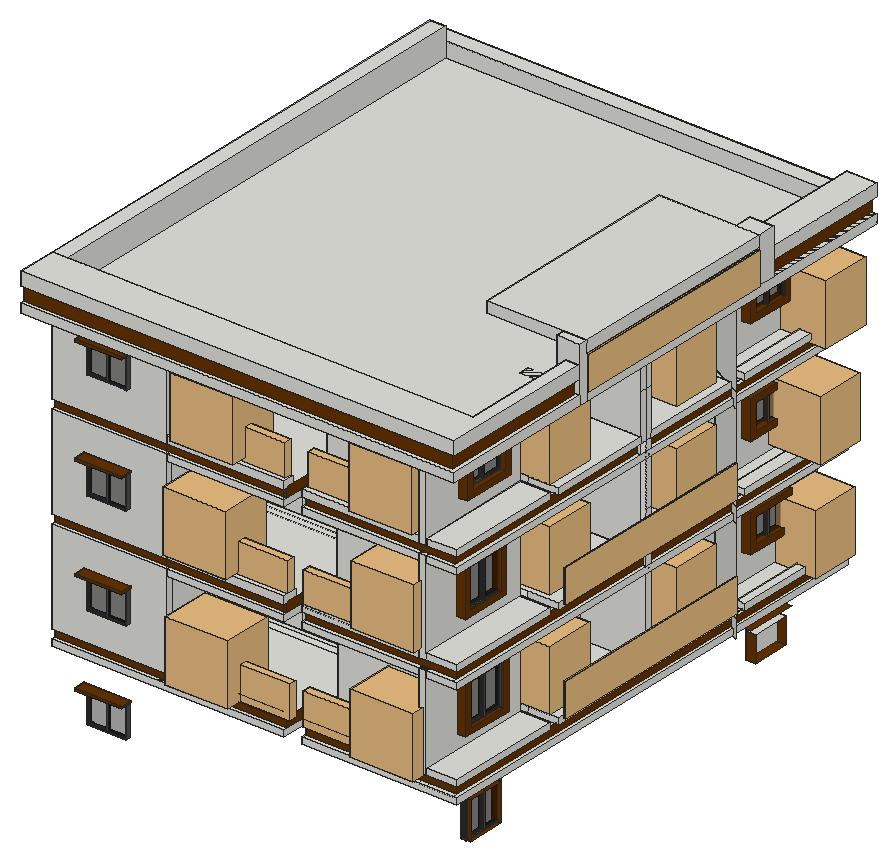
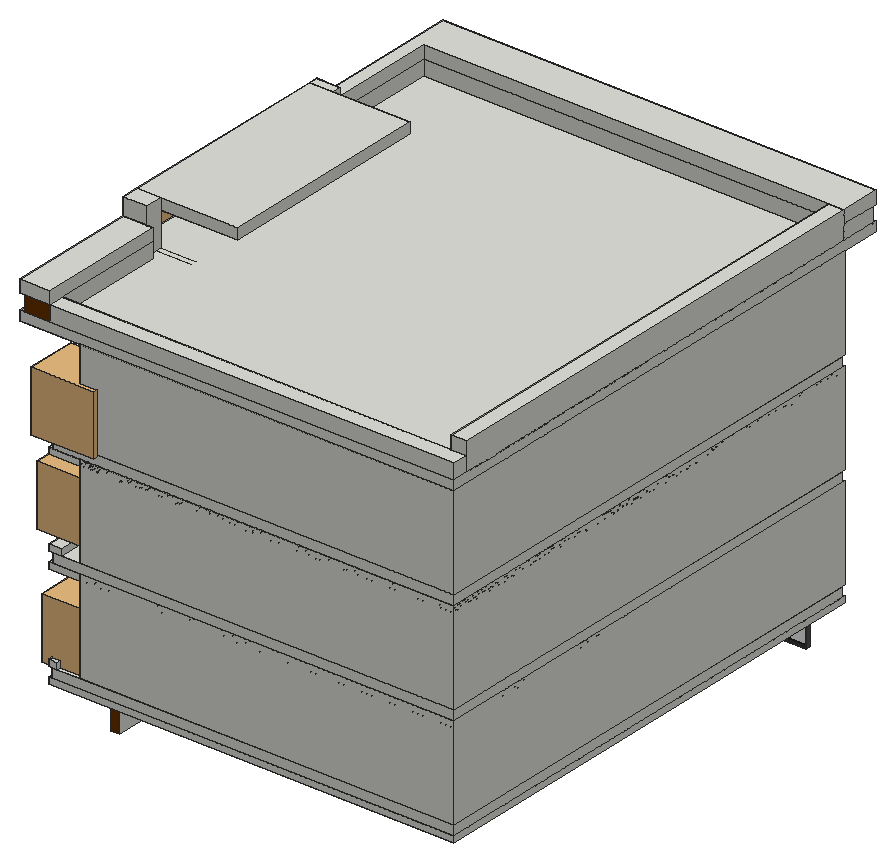
# SketchUp Ruby script. Lengths in inches.
U = 1.inch
M = Sketchup.active_model
def pt(a) = Geom::Point3d.new(a.map { |v| v * U })
def face(e, loops, mat)
  f = e.add_face(loops[0].map { |a| pt(a) })
  loops[1..].each { |l| e.add_face(l.map { |a| pt(a) }).erase! }
  f.material = f.back_material = mat if mat
  f
end
# faces: each face lists its corners as indices into pts; further lists are holes
def faces(e, pts, list, mat = nil) = list.each { |f| face(e, (f[0].is_a?(Array) ? f : [f]).map { |l| l.map { |i| pts[i] } }, mat) }
# xy, xz, yz: faces in a plane at the given z, y or x. An outline is a flat list of corners, or four numbers for a rectangle; further outlines are holes
def ring(l) = l.size == 4 ? [[l[0], l[1]], [l[2], l[1]], [l[2], l[3]], [l[0], l[3]]] : l.each_slice(2).to_a
def flat(e, list, mat, &to3) = list.each { |f| face(e, (f[0].is_a?(Array) ? f : [f]).map { |l| ring(l).map { |u, v| to3.(u, v) } }, mat) }
def xy(e, z, list, mat = nil) = flat(e, list, mat) { |x, y| [x, y, z] }
def xz(e, y, list, mat = nil) = flat(e, list, mat) { |x, z| [x, y, z] }
def yz(e, x, list, mat = nil) = flat(e, list, mat) { |y, z| [x, y, z] }
def lines(e, pts, list) = list.each { |a, b| e.add_line(pt(pts[a]), pt(pts[b])) }
# prism: a flat outline (further loops are holes) pulled along v
def prism(e, loops, v, mat = nil)
  f = face(e, loops, mat); d = Geom::Vector3d.new(v.map { |x| x * U })
  f.pushpull(f.normal.samedirection?(d) ? d.length : -d.length)
end
def box(e, o, s, mat = nil) = prism(e, [[o, [o[0] + s[0], o[1], o[2]], [o[0] + s[0], o[1] + s[1], o[2]], [o[0], o[1] + s[1], o[2]]]], [0, 0, s[2]], mat)
def at(x, y, z, deg = 0) = Geom::Transformation.translation(pt([x, y, z])) * Geom::Transformation.rotation(ORIGIN, Z_AXIS, deg.degrees)
def axes(o, x, y, z) = Geom::Transformation.new([*x, 0, *y, 0, *z, 0, *pt(o).to_a, 1])
def part(name) = M.definitions.add(name)
# library, detail: a bought-in or finely detailed component or shape, given as its bounding box
def library(name, o, s) = part(name).tap { |d| box(d.entities, o, s) }
def detail(e, o, s) = box(e.add_group.entities, o, s)
def put(e, d, t, mat = nil) = e.add_instance(d, t).tap { |i| i.material = mat if mat }
def group(e, t, mat = nil) = e.add_group.tap { |g| g.transformation = t; g.material = mat if mat }.entities
root = M.entities
M.materials.add("Glass_Tinted_Gray").color = [0, 0, 0]
M.materials["Glass_Tinted_Gray"].alpha = 0.125
M.materials.add("[0135_DarkGray]").color = [81, 81, 81]
M.materials.add("[Color C08]").color = [102, 51, 0]
M.materials.add("[Color M00]").color = [255, 255, 255]
M.materials.add("[Mirror 02]").color = [229, 229, 229]
M.materials.add("[Terrazzo Light Blue]").color = [196, 214, 227]
c1 = part("PENTEK_RP Fineline 50S_Sliding_DoorCase_E1")
box(c1.entities,[0,0,0],[1.51,3.66,99.27],"[0135_DarkGray]")
c2 = part("PENTEK_RP Fineline 50S_SlidingDooe_Case_E2")
box(c2.entities,[0,0,0],[96.25,3.66,1.51],"[0135_DarkGray]")
c3 = part("pentek_RP Fineline 50S_SlidingDoor_Case")
put(c3.entities,c1,at(97.76,0,0))
put(c3.entities,c2,at(1.51,0,0))
put(c3.entities,c1,at(0,0,0))
put(c3.entities,c2,at(1.51,0,97.76))
c4 = part("PENTEK_RP Fineline 50S_SlidingDoor_GlazingBead_2")
box(c4.entities,[0,0,0],[0.56,0.59,94.39],"[0135_DarkGray]")
c5 = part("PENTEK_RP Fineline 50S_SlidingDoor_Glass")
box(c5.entities,[0,0,0],[46.58,0.16,94.39],"Glass_Tinted_Gray")
c6 = part("PENTEK_RP Fineline 50S_SlidingDoor_GlazingBead")
box(c6.entities,[0,0,0],[45.47,0.59,0.56],"[0135_DarkGray]")
c7 = part("PENTEK_RP Fineline 50S_SlidingDoor_Leaf_E1")
xy(c7.entities,0,[[0,0,0.93,1.97],[0.93,1.57,1.49,1.97]],"[0135_DarkGray]")
xy(c7.entities,96.25,[[0,0,0.93,0,0.93,1.57,1.49,1.57,1.49,1.97,0,1.97]],"[0135_DarkGray]")
xz(c7.entities,0,[[0,0,0.93,96.25]],"[0135_DarkGray]")
xz(c7.entities,1.57,[[0.93,0,1.49,95.32],[0.93,95.32,1.49,96.25]],"[0135_DarkGray]")
xz(c7.entities,1.97,[[0,0,1.49,96.25]],"[0135_DarkGray]")
yz(c7.entities,0,[[0,0,1.97,96.25]],"[0135_DarkGray]")
yz(c7.entities,0.93,[[0,0,1.57,0.93],[0,0.93,1.57,95.32],[0,95.32,1.57,96.25]],"[0135_DarkGray]")
yz(c7.entities,1.49,[[1.57,0,1.97,95.32],[1.57,95.32,1.97,96.25]],"[0135_DarkGray]")
c8 = part("PENTEK_RP Fineline 50S_SlidingDoor_Leaf_E2")
xy(c8.entities,0,[[0,0,0,1.57,0.56,1.57,0.56,1.97,46.02,1.97,46.02,1.57,46.58,1.57,46.58,0]],"[0135_DarkGray]")
xy(c8.entities,0.93,[[0,0,46.58,1.57]],"[0135_DarkGray]")
xy(c8.entities,1.49,[[0.56,1.57,46.02,1.97]],"[0135_DarkGray]")
xz(c8.entities,0,[[0,0,46.58,0.93]],"[0135_DarkGray]")
xz(c8.entities,1.57,[[0,0,0.56,0.93],[46.02,0,46.58,0.93],[0.56,0.93,46.02,1.49]],"[0135_DarkGray]")
xz(c8.entities,1.97,[[0.56,0,46.02,1.49]],"[0135_DarkGray]")
yz(c8.entities,0,[[0,0,1.57,0.93]],"[0135_DarkGray]")
yz(c8.entities,0.56,[[1.57,0,1.97,0.93],[1.57,0.93,1.97,1.49]],"[0135_DarkGray]")
yz(c8.entities,46.02,[[1.57,0,1.97,0.93],[1.57,0.93,1.97,1.49]],"[0135_DarkGray]")
yz(c8.entities,46.58,[[0,0,1.57,0.93]],"[0135_DarkGray]")
c9 = part("PENTEK_RP Fineline S_SlidingDoor_Leaf1")
put(c9.entities,c4,at(0.93,0,0.93))
put(c9.entities,c4,at(46.96,0,0.93))
put(c9.entities,c5,at(1.49,1.42,0.93))
put(c9.entities,c6,at(1.49,0,0.93))
put(c9.entities,c5,at(1.49,0.59,0.93),"[Terrazzo Light Blue]")
put(c9.entities,c7,at(0,0,0))
put(c9.entities,c7,axes([48.44,0,0],[-1,0,0],[0,1,0],[0,0,1]))
put(c9.entities,c8,axes([0.93,0,96.25],[1,0,0],[0,1,0],[0,0,-1]))
put(c9.entities,c8,at(0.93,0,0))
put(c9.entities,c6,at(1.49,0,94.77))
c10 = part("PENTEK_RP Fineline 50S_SlidingDoor_Leaf2")
put(c10.entities,c5,at(1.49,1.42,0.93))
put(c10.entities,c6,at(1.49,0,94.77))
put(c10.entities,c4,at(46.96,0,0.93))
put(c10.entities,c5,at(1.49,0.59,0.93),"[Mirror 02]")
put(c10.entities,c4,at(0.93,0,0.93))
put(c10.entities,c7,at(0,0,0))
put(c10.entities,c7,axes([48.44,0,0],[-1,0,0],[0,1,0],[0,0,1]))
put(c10.entities,c6,at(1.49,0,0.93))
put(c10.entities,c8,axes([0.93,0,96.25],[1,0,0],[0,1,0],[0,0,-1]))
put(c10.entities,c8,at(0.93,0,0))
c11 = part("PENTEK - Slimmest Steel Sliding Door / Window\#1")
put(c11.entities,c3,at(0,-1.88,-0.09))
put(c11.entities,c9,at(1.51,-2.27,1.42))
put(c11.entities,c10,at(49.32,-0.3,1.42))
c12 = part("Group\#9")
box(c12.entities,[0,0,0],[60.1875,3.0625,15.3125])
c13 = library("Round Planter with Plant",[-35.48,-39.77,0],[80.62,63.55,77.875])
c14 = library("Wagner Glass Railing",[9.08,102.375,1.53],[2.51,145.5,42.05])
xy(root,431.49,[[533.0625,247.82,545.1875,295.73]],"[Color C08]")
xy(root,435.41,[[533.0625,704.34,545.1875,753.42]],"[Color C08]")
xy(root,468.49,[[533.0625,704.34,545.1875,753.42]])
xy(root,476.54,[[533.0625,696.28,545.1875,761.47]],"[Color C08]")
xy(root,479.39,[[533.0625,247.82,545.1875,295.73]],"[Color C08]")
xy(root,486.47,[[533.0625,240.75,545.1875,302.81]],"[Color C08]")
xy(root,507.8125,[[381.78,256.07,524.0625,346.01]])
xy(root,516,[[[53.0625,191.22,200.56,191.22,200.56,346.01,524.0625,346.01,524.0625,191.22,533.0625,191.22,533.0625,355.01,486.8125,355.01,486.8125,495.28,388.3125,495.28,388.3125,502.74,486.8125,502.74,486.8125,631.35,533.0625,631.35,533.0625,818.16,53.0625,818.16],[62.0625,200.22,62.0625,809.84,524.0625,809.84,524.0625,640.35,379.3125,640.35,379.3125,355.01,191.56,355.01,191.56,200.22]]])
xy(root,528,[[[53.0625,191.22,200.56,191.22,200.56,346.01,383.92,346.01,383.92,236.51,524.0625,236.51,524.0625,191.22,532.86,191.22,532.86,341.375,533.0625,341.375,533.0625,355.01,388.3125,355.01,388.3125,631.35,533.0625,631.35,533.0625,818.16,53.0625,818.16],[62.0625,200.22,62.0625,809.84,524.0625,809.84,524.0625,640.35,379.3125,640.35,379.3125,355.01,191.56,355.01,191.56,200.22]],[532.86,191.22,533.0625,341.375],[62.0625,200.22,191.56,200.22,191.56,355.01,379.3125,355.01,379.3125,640.35,524.0625,640.35,524.0625,809.84,62.0625,809.84],[388.3125,495.28,572.25,502.74],[533.0625,641.54,572.25,641.54,572.25,653.47,561.5,653.47,561.5,818.16,533.0625,818.16]])
xy(root,535.4375,[[388.3125,355.01,486.8125,495.28],[486.8125,355.01,572.25,495.28],[388.3125,502.74,486.8125,631.35],[486.8125,502.74,572.25,631.35]])
xy(root,536.1875,[[532.86,191.22,572.25,341.375],[561.5,653.47,572.25,818.16]])
xy(root,554.18,[[533.0625,240.52,545.1875,308.45]])
xy(root,561.26,[[533.0625,247.59,545.1875,301.375]],"[Color C08]")
xy(root,563.11,[[533.0625,696.28,545.1875,761.47]],"[Color C08]")
xy(root,571.16,[[533.0625,704.34,545.1875,753.42]],"[Color C08]")
xy(root,604.24,[[533.0625,704.34,545.1875,753.42]])
xy(root,612.29,[[533.0625,696.28,545.1875,761.47]],"[Color C08]")
xy(root,615.03,[[533.0625,247.59,545.1875,301.375]],"[Color C08]")
xy(root,622.11,[[533.0625,240.52,545.1875,308.45]],"[Color C08]")
xy(root,639.8125,[[383.92,236.51,524.0625,346.01]])
xy(root,648,[[[53.0625,191.22,200.56,191.22,200.56,346.01,524.0625,346.01,524.0625,191.22,533.0625,191.22,533.0625,355.01,486.8125,355.01,486.8125,495.28,388.3125,495.28,388.3125,502.74,486.8125,502.74,486.8125,631.35,533.0625,631.35,533.0625,818.16,53.0625,818.16],[62.0625,200.22,62.0625,809.84,524.0625,809.84,524.0625,640.35,379.3125,640.35,379.3125,355.01,191.56,355.01,191.56,200.22]]])
xy(root,660,[[[53.0625,191.22,200.56,191.22,200.56,346.01,372.32,346.01,372.32,248.7,524.0625,248.7,524.0625,191.22,533.0625,191.22,533.0625,355.01,388.3125,355.01,388.3125,631.35,533.0625,631.35,533.0625,818.16,53.0625,818.16],[62.0625,200.22,62.0625,809.84,524.0625,809.84,524.0625,640.35,379.3125,640.35,379.3125,355.01,191.56,355.01,191.56,200.22]],[62.0625,200.22,191.56,200.22,191.56,355.01,379.3125,355.01,379.3125,640.35,524.0625,640.35,524.0625,809.84,62.0625,809.84],[388.3125,355.01,572.25,487.09],[388.3125,487.09,572.25,495.28],[388.3125,495.28,572.25,502.74],
  [533.0625,641.54,572.25,641.54,572.25,653.47,555.82,653.47,555.82,818.16,533.0625,818.16]])
xy(root,668.1875,[[533.0625,191.22,572.25,341.375],[486.8125,355.01,572.25,487.09],[388.3125,502.74,486.8125,631.35],[486.8125,502.74,572.25,631.35],[555.82,653.47,572.25,818.16]])
xy(root,669.4375,[[200.56,191.22,350.31,211.34],[374.31,191.22,524.0625,208.91]])
xy(root,689.44,[[533.0625,239.83,545.1875,304.08]],"[Color C08]")
xy(root,693.73,[[533.0625,696.28,545.1875,761.47]],"[Color C08]")
xy(root,696.52,[[533.0625,246.91,545.1875,297]],"[Color C08]")
xy(root,701.79,[[533.0625,704.34,545.1875,753.42]],"[Color C08]")
xy(root,734.86,[[533.0625,704.34,545.1875,753.42]])
xy(root,742.92,[[533.0625,696.28,545.1875,761.47]],"[Color C08]")
xy(root,746.61,[[533.0625,246.91,545.1875,297]],"[Color C08]")
xy(root,753.69,[[533.0625,239.83,545.1875,304.08]],"[Color C08]")
xy(root,771.8125,[[372.32,248.7,524.0625,346.01]])
xy(root,780,[[[53.0625,191.22,200.56,191.22,200.56,346.01,524.0625,346.01,524.0625,191.22,533.0625,191.22,533.0625,355.01,486.8125,355.01,486.8125,487.09,388.3125,487.09,388.3125,502.74,486.8125,502.74,486.8125,631.35,533.0625,631.35,533.0625,818.16,53.0625,818.16],[62.0625,200.22,62.0625,809.84,524.0625,809.84,524.0625,640.35,379.3125,640.35,379.3125,355.01,191.56,355.01,191.56,200.22]]])
xy(root,792,[[[53.0625,191.22,200.56,191.22,200.56,346.01,352.68,346.01,352.68,257.47,524.0625,257.47,524.0625,191.22,533.0625,191.22,533.0625,355.01,388.3125,355.01,388.3125,631.35,533.0625,631.35,533.0625,818.16,53.0625,818.16],[62.0625,200.22,62.0625,809.84,524.0625,809.84,524.0625,640.35,379.3125,640.35,379.3125,355.01,191.56,355.01,191.56,200.22]],[533.0625,191.22,533.65,341.375],[62.0625,200.22,191.56,200.22,191.56,355.01,379.3125,355.01,379.3125,640.35,524.0625,640.35,524.0625,809.84,62.0625,809.84],[200.56,205.69,350.31,205.69,350.31,232.22,352.68,232.22,352.68,346.01,200.56,346.01],[374.31,211.34,524.0625,257.47],
  [388.3125,355.01,572.25,487.09],[388.3125,487.09,572.25,502.74],[533.0625,641.54,572.25,641.54,572.25,653.47,557.85,653.47,557.85,818.16,533.0625,818.16]])
xy(root,800.1875,[[533.65,191.22,572.25,341.375],[388.3125,355.01,486.8125,487.09],[486.8125,355.01,572.25,487.09],[388.3125,502.74,486.8125,631.35],[486.8125,502.74,572.25,631.35],
  [557.85,653.47,572.25,818.16]])
xy(root,801.4375,[[200.56,191.22,350.31,205.69],[374.31,191.22,524.0625,211.34]])
xy(root,824.5,[[533.0625,242.66,545.1875,311.73]],"[Color C08]")
xy(root,828.29,[[533.0625,696.28,545.1875,761.47]],"[Color C08]")
xy(root,832.35,[[533.0625,250.51,545.1875,303.88]],"[Color C08]")
xy(root,836.35,[[533.0625,704.34,545.1875,753.42]],"[Color C08]")
xy(root,869.43,[[533.0625,704.34,545.1875,753.42]])
xy(root,877.48,[[533.0625,696.28,545.1875,761.47]],"[Color C08]")
xy(root,885.71,[[533.0625,250.51,545.1875,303.88]],"[Color C08]")
xy(root,893.5625,[[533.0625,242.66,545.1875,311.73]],"[Color C08]")
xy(root,910.375,[[388.3125,487.09,486.8125,502.74],[486.8125,487.09,572.25,502.74]])
xy(root,912,[[352.68,257.47,524.0625,346.01]])
xy(root,924,[[53.0625,146.72,53.0625,193.17,592.21,193.17,592.21,340.92,603.25,340.92,603.25,146.72],[533.0625,341.375,578.3125,355.01],[578.3125,631.35,608.75,653.47],[602.625,653.47,608.75,818.16]])
xy(root,943.375,[[53.0625,141.41,608.75,146.72],[53.0625,146.72,53.0625,193.17,592.21,193.17,592.21,340.92,603.25,340.92,603.25,146.72],[603.25,146.72,608.75,340.92],[570.58,653.47,602.625,818.16],[602.625,653.47,608.75,818.16],
  [53.0625,797.98,570.58,818.16]])
xy(root,959.875,[[53.0625,141.41,608.75,141.41,608.75,340.92,592.21,340.92,592.21,193.17,53.0625,193.17],[53.0625,193.17,72.8,797.98],[570.58,653.47,608.75,818.16]])
xy(root,967.8,[[479.8125,355.01,608.75,631.35]])
xy(root,982.0625,[[479.8125,355.01,608.75,631.35],[578.3125,631.35,608.75,653.47]])
xz(root,141.41,[[53.0625,943.375,608.75,959.875]])
xz(root,146.72,[[53.0625,924,603.25,943.375]],"[Color C08]")
xz(root,191.22,[[53.0625,528,200.56,648],[524.0625,528,532.86,528,532.86,536.1875,533.0625,536.1875,533.0625,648,524.0625,648],[532.86,528,533.0625,536.1875],[533.0625,528,572.25,536.1875],[53.0625,660,200.56,780],
  [200.56,660,350.31,669.4375],[374.31,660,524.0625,669.4375],[524.0625,660,533.0625,780],[533.0625,660,572.25,668.1875],[53.0625,792,200.56,912],
  [200.56,792,350.31,801.4375],[374.31,792,524.0625,801.4375],[524.0625,792,533.0625,912],[533.65,792,572.25,800.1875]])
xz(root,193.17,[[53.0625,924,72.8,943.375],[72.8,924,592.21,943.375],[53.0625,943.375,72.8,959.875],[72.8,943.375,592.21,959.875]])
xz(root,200.22,[[62.0625,528,191.56,648],[62.0625,660,191.56,780],[62.0625,792,191.56,912]])
xz(root,205.69,[[200.56,792,350.31,801.4375]])
xz(root,208.91,[[374.31,660,524.0625,669.4375]])
xz(root,211.34,[[200.56,660,350.31,669.4375],[374.31,792,524.0625,801.4375]])
xz(root,236.51,[[383.92,528,524.0625,639.8125]])
xz(root,239.83,[[533.0625,689.44,545.1875,753.69]],"[Color C08]")
xz(root,240.52,[[533.0625,554.18,545.1875,622.11]],"[Color C08]")
xz(root,242.66,[[533.0625,824.5,545.1875,893.5625]],"[Color C08]")
xz(root,246.91,[[533.0625,696.52,545.1875,746.61]],"[Color C08]")
xz(root,247.59,[[533.0625,561.26,545.1875,615.03]],"[Color C08]")
xz(root,247.82,[[533.0625,431.49,545.1875,479.39]],"[Color C08]")
xz(root,248.7,[[372.32,660,524.0625,771.8125]])
xz(root,250.51,[[533.0625,832.35,545.1875,885.71]],"[Color C08]")
xz(root,257.47,[[352.68,792,524.0625,912]])
xz(root,295.73,[[533.0625,431.49,545.1875,479.39]],"[Color C08]")
xz(root,297,[[533.0625,696.52,545.1875,746.61]],"[Color C08]")
xz(root,301.375,[[533.0625,561.26,545.1875,615.03]],"[Color C08]")
xz(root,303.88,[[533.0625,832.35,545.1875,885.71]],"[Color C08]")
xz(root,304.08,[[533.0625,689.44,545.1875,753.69]],"[Color C08]")
xz(root,308.45,[[533.0625,554.18,545.1875,622.11]],"[Color C08]")
xz(root,311.73,[[533.0625,824.5,545.1875,893.5625]],"[Color C08]")
xz(root,340.92,[[592.21,924,603.25,943.375],[592.21,943.375,608.75,959.875]])
xz(root,341.375,[[532.86,528,533.0625,536.1875],[533.0625,528,572.25,536.1875],[533.0625,660,572.25,668.1875],[533.65,792,572.25,800.1875]])
xz(root,346.01,[[200.56,528,383.92,528,383.92,639.8125,524.0625,639.8125,524.0625,648,200.56,648],[200.56,660,372.32,660,372.32,771.8125,524.0625,771.8125,524.0625,780,200.56,780],[200.56,792,352.68,912]])
xz(root,355.01,[[191.56,528,379.3125,648],[388.3125,528,533.0625,535.4375],[533.0625,528,572.25,535.4375],[191.56,660,379.3125,780],[533.0625,660,572.25,668.1875],
  [191.56,792,379.3125,912],[388.3125,792,533.0625,800.1875],[533.0625,792,572.25,800.1875],[479.8125,967.8,608.75,982.0625]])
xz(root,487.09,[[388.3125,660,572.25,668.1875],[388.3125,668.1875,486.8125,780],[486.8125,668.1875,572.25,668.1875,572.25,792,388.3125,792,388.3125,780,486.8125,780],[388.3125,792,572.25,800.1875],[388.3125,800.1875,486.8125,910.375],
  [486.8125,800.1875,572.25,910.375]])
xz(root,495.28,[[388.3125,528,572.25,535.4375],[388.3125,535.4375,486.8125,648],[486.8125,535.4375,572.25,535.4375,572.25,660,388.3125,660,388.3125,648,486.8125,648]])
xz(root,502.74,[[388.3125,528,572.25,535.4375],[388.3125,535.4375,486.8125,648],[486.8125,535.4375,486.8125,648,388.3125,648,388.3125,660,572.25,660,572.25,535.4375],[388.3125,660,572.25,668.1875],[388.3125,668.1875,486.8125,780],
  [486.8125,668.1875,486.8125,780,388.3125,780,388.3125,792,572.25,792,572.25,668.1875],[388.3125,792,572.25,800.1875],[388.3125,800.1875,486.8125,910.375],[486.8125,800.1875,572.25,910.375]])
xz(root,631.35,[[388.3125,528,533.0625,535.4375],[533.0625,528,572.25,535.4375],[388.3125,660,533.0625,668.1875],[533.0625,660,572.25,668.1875],[388.3125,792,533.0625,800.1875],
  [533.0625,792,572.25,800.1875],[578.3125,924,608.75,967.8],[479.8125,967.8,578.3125,982.0625]])
xz(root,640.35,[[379.3125,528,524.0625,648],[379.3125,660,524.0625,780],[379.3125,792,524.0625,912]])
xz(root,653.47,[[561.5,528,572.25,536.1875],[555.82,660,572.25,668.1875],[557.85,792,572.25,800.1875],[578.3125,924,602.625,943.375],[602.625,924,608.75,943.375],
  [570.58,943.375,578.3125,959.875],[578.3125,943.375,608.75,959.875],[578.3125,959.875,608.75,982.0625]])
xz(root,696.28,[[533.0625,563.11,545.1875,612.29],[533.0625,693.73,545.1875,742.92],[533.0625,828.29,545.1875,877.48]],"[Color C08]")
xz(root,704.34,[[533.0625,435.41,545.1875,468.49],[533.0625,571.16,545.1875,604.24],[533.0625,701.79,545.1875,734.86],[533.0625,836.35,545.1875,869.43]],"[Color C08]")
xz(root,753.42,[[533.0625,435.41,545.1875,468.49],[533.0625,571.16,545.1875,604.24],[533.0625,701.79,545.1875,734.86],[533.0625,836.35,545.1875,869.43]],"[Color C08]")
xz(root,761.47,[[533.0625,563.11,545.1875,612.29],[533.0625,693.73,545.1875,742.92],[533.0625,828.29,545.1875,877.48]],"[Color C08]")
xz(root,797.98,[[72.8,924,570.58,943.375],[53.0625,943.375,72.8,959.875]])
xz(root,809.84,[[62.0625,528,524.0625,648],[62.0625,660,524.0625,780],[62.0625,792,524.0625,912]])
xz(root,818.16,[[53.0625,528,533.0625,648],[561.5,528,572.25,536.1875],[53.0625,660,533.0625,780],[555.82,660,572.25,668.1875],[53.0625,792,533.0625,912],
  [557.85,792,572.25,800.1875],[53.0625,924,570.58,943.375],[570.58,943.375,608.75,959.875]])
xz(root,818.16,[[570.58,924,602.625,943.375]],"[Color C08]")
yz(root,53.0625,[[191.22,528,818.16,648],[191.22,660,818.16,780],[191.22,792,818.16,912],[146.72,924,193.17,943.375],[193.17,924,797.98,959.875],
  [797.98,924,818.16,943.375],[141.41,943.375,193.17,959.875]])
yz(root,62.0625,[[200.22,528,809.84,648],[200.22,660,809.84,780],[200.22,792,809.84,912]])
yz(root,72.8,[[193.17,924,797.98,959.875]])
yz(root,191.56,[[200.22,528,355.01,648],[200.22,660,355.01,780],[200.22,792,355.01,912]])
yz(root,200.56,[[191.22,528,199.58,537.4375],[199.58,528,200.22,528,200.22,648,191.22,648,191.22,537.4375,199.58,537.4375],[200.22,528,346.01,648],[191.22,660,200.22,669.4375],[200.22,660,211.34,669.4375],
  [211.34,660,346.01,660,346.01,780,200.22,780,200.22,669.4375,211.34,669.4375],[191.22,669.4375,200.22,780],[191.22,792,200.22,801.4375],[200.22,792,205.69,801.4375],[205.69,792,346.01,792,346.01,912,200.22,912,200.22,801.4375,205.69,801.4375],
  [191.22,801.4375,200.22,912]])
yz(root,350.31,[[191.22,660,211.34,669.4375],[191.22,792,205.69,801.4375]])
yz(root,352.68,[[257.47,792,346.01,912]])
yz(root,372.32,[[248.7,660,346.01,771.8125]])
yz(root,374.31,[[191.22,660,208.91,669.4375],[191.22,792,211.34,801.4375]])
yz(root,379.3125,[[355.01,528,640.35,648],[355.01,660,640.35,780],[355.01,792,640.35,912]])
yz(root,383.92,[[236.51,528,346.01,639.8125]])
yz(root,388.3125,[[495.28,516,502.74,528],[355.01,528,495.28,535.4375],[495.28,528,502.74,648],[502.74,528,631.35,535.4375],[495.28,648,502.74,660],
  [355.01,660,487.09,668.1875],[487.09,660,502.74,780],[502.74,660,631.35,668.1875],[487.09,780,502.74,792],[355.01,792,487.09,800.1875],
  [487.09,792,502.74,910.375],[502.74,792,631.35,800.1875]])
yz(root,479.8125,[[355.01,967.8,631.35,982.0625]])
yz(root,486.8125,[[355.01,535.4375,495.28,648],[502.74,535.4375,631.35,648],[355.01,668.1875,487.09,780],[502.74,668.1875,631.35,780],[355.01,800.1875,487.09,800.1875,487.09,910.375,502.74,910.375,502.74,800.1875,631.35,800.1875,631.35,912,355.01,912]])
yz(root,524.0625,[[191.22,528,200.22,537.4375],[200.22,528,200.22,648,346.01,648,346.01,639.8125,236.51,639.8125,236.51,528],[640.35,528,809.84,648],[191.22,537.4375,200.22,648],[191.22,660,200.22,669.4375],
  [200.22,660,208.91,669.4375],[208.91,660,208.91,669.4375,200.22,669.4375,200.22,780,346.01,780,346.01,771.8125,248.7,771.8125,248.7,660],[248.7,660,346.01,771.8125],[640.35,660,809.84,780],[191.22,669.4375,200.22,780],
  [191.22,792,200.22,801.4375],[200.22,792,211.34,801.4375],[211.34,792,211.34,801.4375,200.22,801.4375,200.22,912,257.47,912,257.47,792],[640.35,792,809.84,912],[191.22,801.4375,200.22,912]])
yz(root,532.86,[[191.22,528,341.375,536.1875]])
yz(root,533.0625,[[247.82,431.49,295.73,479.39],[704.34,435.41,753.42,468.49],[341.375,516,355.01,528],[631.35,516,653.47,528],[[191.22,528,341.375,648],[240.52,554.18,308.45,622.11]],
  [[653.47,528,818.16,648],[696.28,563.11,761.47,612.29]],[247.59,561.26,301.375,615.03],[704.34,571.16,753.42,604.24],[341.375,648,355.01,660],[631.35,648,653.47,660],
  [[653.47,660,818.16,780],[696.28,693.73,761.47,742.92]],[[191.22,668.1875,341.375,780],[239.83,689.44,304.08,753.69]],[246.91,696.52,297,746.61],[704.34,701.79,753.42,734.86],[341.375,780,355.01,792],
  [631.35,780,653.47,792],[[191.22,792,341.375,912],[242.66,824.5,311.73,893.5625]],[[653.47,792,818.16,912],[696.28,828.29,761.47,877.48]],[250.51,832.35,303.88,885.71],[704.34,836.35,753.42,869.43],
  [341.375,912,355.01,924]])
yz(root,533.65,[[191.22,792,341.375,800.1875]])
yz(root,545.1875,[[[240.52,554.18,308.45,622.11],[247.59,561.26,301.375,615.03]],[[696.28,563.11,761.47,612.29],[704.34,571.16,753.42,604.24]],[[239.83,689.44,304.08,753.69],[246.91,696.52,297,746.61]],[[696.28,693.73,761.47,742.92],[704.34,701.79,753.42,734.86]],[[242.66,824.5,311.73,893.5625],[250.51,832.35,303.88,885.71]],
  [[696.28,828.29,761.47,877.48],[704.34,836.35,753.42,869.43]]],"[Color C08]")
yz(root,555.82,[[653.47,660,818.16,668.1875]])
yz(root,557.85,[[653.47,792,818.16,800.1875]])
yz(root,561.5,[[653.47,528,818.16,536.1875]])
yz(root,570.58,[[653.47,924,797.98,943.375],[653.47,943.375,818.16,959.875]])
yz(root,572.25,[[191.22,528,341.375,536.1875],[355.01,528,495.28,535.4375],[495.28,528,502.74,660],[502.74,528,631.35,535.4375],[653.47,528,818.16,536.1875],
  [191.22,660,341.375,668.1875],[355.01,660,487.09,668.1875],[495.28,660,502.74,712.8125],[502.74,660,631.35,668.1875],[653.47,660,818.16,668.1875],
  [495.28,712.8125,502.74,792],[191.22,792,341.375,800.1875],[355.01,792,487.09,800.1875],[487.09,792,495.28,852.4375],[495.28,792,502.74,852.4375],
  [502.74,792,631.35,800.1875],[653.47,792,818.16,800.1875],[487.09,852.4375,495.28,910.375],[495.28,852.4375,502.74,910.375]])
yz(root,572.25,[[487.09,660,495.28,792]],"[Color M00]")
yz(root,578.3125,[[631.35,924,653.47,982.0625]])
yz(root,592.21,[[193.17,924,340.92,943.375],[193.17,943.375,340.92,959.875]])
yz(root,602.625,[[653.47,924,818.16,943.375]],"[Color C08]")
yz(root,603.25,[[146.72,924,340.92,943.375]],"[Color C08]")
yz(root,608.75,[[631.35,924,653.47,982.0625],[141.41,943.375,340.92,959.875],[653.47,943.375,818.16,959.875],[355.01,967.8,631.35,982.0625]])
p = [[578.3125,631.35,530.96],[533.0625,653.47,530.96],[533.0625,653.47,528],[533.0625,653.47,516],[533.0625,653.47,507.8125],[578.3125,631.35,507.8125],
  [578.3125,631.35,639.8125],[533.0625,653.47,639.8125],[578.3125,631.35,660.1875],[533.0625,653.47,660.1875],[533.0625,653.47,660],[533.0625,653.47,648],
  [379.3125,355.01,660],[524.0625,346.01,660],[524.0625,346.01,771.8125],[379.3125,355.01,771.8125],[578.3125,631.35,771.8125],[533.0625,653.47,771.8125],
  [578.3125,631.35,791.43],[533.0625,653.47,791.43],[533.0625,653.47,780],[533.0625,653.47,912],[533.0625,653.47,792],[578.3125,631.35,912],
  [350.31,232.22,528],[374.31,232.22,528],[350.31,191.22,660],[350.31,191.22,648],[374.31,191.22,660],[374.31,191.22,648],
  [374.31,191.22,792],[374.31,191.22,780],[350.31,191.22,792],[350.31,191.22,780],[200.56,191.22,528],[200.56,191.22,516],
  [200.56,191.22,660],[200.56,191.22,648],[200.56,191.22,792],[200.56,191.22,780],[350.31,191.22,528],[350.31,199.58,528],
  [200.56,199.58,528],[374.31,191.22,528],[524.0625,191.22,528],[524.0625,200.22,528],[374.31,200.22,528],[524.0625,200.22,537.4375],
  [374.31,200.22,537.4375],[374.31,191.22,537.4375],[524.0625,191.22,537.4375],[350.31,199.58,537.4375],[200.56,199.58,537.4375],[200.56,191.22,537.4375],
  [350.31,191.22,537.4375],[350.31,211.34,660],[350.31,232.22,660],[374.31,208.91,660],[374.31,232.22,660],[578.3125,341.375,912],
  [608.75,343.9375,912],[578.3125,355.01,912],[608.75,355.01,912],[608.75,343.9375,924],[608.75,355.01,924],[583.8125,343.9375,924],
  [583.8125,355.01,924],[578.3125,631.35,924],[533.0625,631.35,924],[578.3125,638.54,924],[533.0625,638.54,924],[533.0625,631.35,912]]
faces(root,p,[[0,1,2,3,4,5],[1,0,6,7],[8,9,10,11,7,6],[12,13,14,15],[9,8,16,17],[18,19,20,17,16],[21,22,19,18,23]])
lines(root,p,[[24,25],[26,27],[28,29],[30,31],[32,33],[34,35],[36,37],[38,39],[34,40],[41,42],[41,24],[43,44],
  [45,46],[47,48],[49,50],[51,52],[53,54],[55,56],[57,58],[59,60],[61,62],[60,63],[62,64],[63,65],
  [64,66],[67,68],[69,70],[71,21]])
put(root,c11,axes([538.74,300.23,432.15],[0,-0.5528,0],[-1.51244,0,0],[0,0,0.5307]))
put(root,c11,axes([153.96,188.68,437.68],[-0.51717,0,0],[0,1.4209,0],[0,0,0.41395]))
put(root,c12,axes([95.21,191.22,478.14],[1,0,0],[0,0,1],[0,-1,0]),"[Color C08]")
g1 = group(root,at(53.0625,818.16,516))
xy(g1,-8.1875,[[0,-626.9375,0,0,519.1875,0,519.1875,-626.9375,321.25,-626.9375,321.25,-586.6875,297.25,-586.6875,297.25,-626.9375]])
xy(g1,0,[[0,-626.9375,297.25,-621.1875],[321.25,-626.9375,515,-621.1875],[515,-626.9375,519.1875,0],[0,-621.1875,297.25,-621.1875,297.25,-586.6875,321.25,-586.6875,321.25,-621.1875,515,-621.1875,515,0,0,0]])
xz(g1,-626.9375,[[0,-8.1875,297.25,0],[321.25,-8.1875,519.1875,0]])
xz(g1,-621.1875,[[0,0,297.25,12],[321.25,0,515,12]],"[Color C08]")
xz(g1,-586.6875,[[297.25,-8.1875,321.25,0]])
xz(g1,-586.6875,[[297.25,0,321.25,12]],"[Color C08]")
xz(g1,0,[[0,-8.1875,519.1875,0],[0,0,515,12]])
yz(g1,0,[[-626.9375,-8.1875,0,0],[-621.1875,0,0,12]])
yz(g1,297.25,[[-626.9375,-8.1875,-586.6875,0]])
yz(g1,297.25,[[-621.1875,0,-586.6875,12]],"[Color C08]")
yz(g1,321.25,[[-626.9375,-8.1875,-586.6875,0]])
yz(g1,321.25,[[-621.1875,0,-586.6875,12]],"[Color C08]")
yz(g1,515,[[-621.1875,0,0,12]],"[Color C08]")
yz(g1,519.1875,[[-626.9375,-8.1875,0,0]])
put(root,c13,at(247.01,215.21,526.26))
put(root,c13,at(484.19,215.21,526.26))
put(root,c13,at(540.42,789.45,526.58))
put(root,c14,axes([90.56,158.16,525.99],[0,3.9,0],[1.07184,0,0],[0,0,1]))
put(root,c14,axes([271.66,155.82,526.45],[0,3.9,0],[1.01825,0,0],[0,0,1]))
put(root,c13,at(515.72,394.78,535.77))
put(root,c14,axes([567.64,165.71,534.55],[1,0,0],[0,1.88042,0],[0,0,1]))
put(root,c13,at(515.28,598.17,536.33))
put(root,c11,axes([538.74,300.23,562.27],[0,-0.5528,0],[-1.51244,0,0],[0,0,0.5307]),"[Color C08]")
put(root,c11,axes([538.58,754.625,564.24],[0,-0.51717,0],[-1.4209,0,0],[0,0,0.41395]))
put(root,c11,axes([153.96,188.68,568.68],[-0.51717,0,0],[0,1.4209,0],[0,0,0.41395]))
put(root,c12,axes([95.21,191.22,609.45],[1,0,0],[0,0,1],[0,-1,0]),"[Color C08]")
g2 = group(root,at(53.0625,818.16,648))
xy(g2,-8.1875,[[0,-626.9375,0,0,519.1875,0,519.1875,-626.9375,321.25,-626.9375,321.25,-586.6875,297.25,-586.6875,297.25,-626.9375]])
xy(g2,0,[[0,-626.9375,297.25,-621.1875],[321.25,-626.9375,514.375,-621.1875],[514.375,-626.9375,519.1875,0],[0,-621.1875,297.25,-621.1875,297.25,-586.6875,321.25,-586.6875,321.25,-621.1875,514.375,-621.1875,514.375,0,0,0]])
xz(g2,-626.9375,[[0,-8.1875,297.25,0],[321.25,-8.1875,519.1875,0]])
xz(g2,-621.1875,[[0,0,297.25,12],[321.25,0,514.375,12]],"[Color C08]")
xz(g2,-586.6875,[[297.25,-8.1875,321.25,0],[297.25,0,321.25,12]])
xz(g2,0,[[0,-8.1875,519.1875,0],[0,0,514.375,12]])
yz(g2,0,[[-626.9375,-8.1875,0,0],[-621.1875,0,0,12]])
yz(g2,297.25,[[-626.9375,-8.1875,-586.6875,0]])
yz(g2,297.25,[[-621.1875,0,-586.6875,12]],"[Color C08]")
yz(g2,321.25,[[-626.9375,-8.1875,-586.6875,0]])
yz(g2,321.25,[[-621.1875,0,-586.6875,12]],"[Color C08]")
yz(g2,514.375,[[-621.1875,0,0,12]],"[Color C08]")
yz(g2,519.1875,[[-626.9375,-8.1875,0,0]])
put(root,c14,axes([94.95,162.87,663.57],[0,3.9,0],[1.02897,0,0],[0,0,1]))
put(root,c14,axes([567.49,165.71,665.12],[1,0,0],[0,1.88042,0],[0,0,1]))
put(root,c14,axes([271.66,155.82,665.14],[0,3.9,0],[1.01825,0,0],[0,0,1]))
put(root,c13,at(555.82,777.96,668.1875))
put(root,c13,at(241.01,219.5625,671.16))
put(root,c13,at(481.32,219.5625,671.16))
put(root,c13,at(515.72,394.78,672.71))
put(root,c13,at(515.28,598.17,673.26))
put(root,c11,axes([538.58,754.625,694.87],[0,-0.51717,0],[-1.4209,0,0],[0,0,0.41395]))
put(root,c11,axes([538.74,300.23,695.77],[0,-0.5528,0],[-1.51244,0,0],[0,0,0.5307]),"[Color C08]")
put(root,c11,axes([153.96,188.68,700.36],[-0.51717,0,0],[0,1.4209,0],[0,0,0.41395]))
put(root,c12,axes([95.21,191.22,742.08],[1,0,0],[0,0,1],[0,-1,0]),"[Color C08]")
g3 = group(root,at(53.0625,818.16,780))
xy(g3,-8.1875,[[0,-626.9375,0,0,519.1875,0,519.1875,-626.9375,321.25,-626.9375,321.25,-586.6875,297.25,-586.6875,297.25,-626.9375]])
xy(g3,0,[[0,-626.9375,297.25,-621.1875],[321.25,-626.9375,513.75,-621.1875],[513.75,-626.9375,519.1875,0],[0,-621.1875,297.25,-621.1875,297.25,-586.6875,321.25,-586.6875,321.25,-621.1875,513.75,-621.1875,513.75,0,0,0]])
xz(g3,-626.9375,[[0,-8.1875,297.25,0],[321.25,-8.1875,519.1875,0]])
xz(g3,-621.1875,[[0,0,297.25,12],[321.25,0,513.75,12]],"[Color C08]")
xz(g3,-586.6875,[[297.25,-8.1875,321.25,0]])
xz(g3,-586.6875,[[297.25,0,321.25,12]],"[Color C08]")
xz(g3,0,[[0,-8.1875,519.1875,0],[0,0,513.75,12]])
yz(g3,0,[[-626.9375,-8.1875,0,0],[-621.1875,0,0,12]])
yz(g3,297.25,[[-626.9375,-8.1875,-586.6875,0]])
yz(g3,297.25,[[-621.1875,0,-586.6875,12]],"[Color C08]")
yz(g3,321.25,[[-626.9375,-8.1875,-586.6875,0]])
yz(g3,321.25,[[-621.1875,0,-586.6875,12]],"[Color C08]")
yz(g3,513.75,[[-621.1875,0,0,12]],"[Color C08]")
yz(g3,519.1875,[[-626.9375,-8.1875,0,0]])
put(root,c13,at(546.59,798.42,788.81))
put(root,c13,at(515.72,394.78,798.96))
put(root,c14,axes([97.14,162.87,797.82],[0,3.9,0],[1.00753,0,0],[0,0,1]))
put(root,c14,axes([271.93,162.87,797.82],[0,3.9,0],[1.01825,0,0],[0,0,1]))
put(root,c13,at(515.28,598.17,799.51))
put(root,c13,at(249.6,219.59,805.42))
put(root,c13,at(478.35,219.59,805.42))
put(root,c11,axes([538.58,754.625,829.43],[0,-0.51717,0],[-1.4209,0,0],[0,0,0.41395]))
put(root,c11,axes([535.25,303.88,833.08],[0,-0.5528,0],[-1.51244,0,0],[0,0,0.5307]))
put(root,c11,axes([153.96,188.85,839.05],[-0.51717,0,0],[0,1.4209,0],[0,0,0.41395]))
put(root,c12,axes([95.21,191.22,878.87],[1,0,0],[0,0,1],[0,-1,0]),"[Color C08]")
g4 = group(root,at(53.0625,818.16,912))
xy(g4,0,[[0,-676.75,555.6875,0]])
xy(g4,12,[[0,-676.75,555.6875,-676.75,555.6875,-474.22,525.25,-474.22,525.25,-463.15,555.6875,-463.15,555.6875,0,0,0]])
xy(g4,70.0625,[[525.25,-474.22,555.6875,-463.15]])
xz(g4,-676.75,[[0,0,555.6875,12]])
xz(g4,-474.22,[[525.25,12,555.6875,70.0625]])
xz(g4,-463.15,[[525.25,12,555.6875,70.0625]])
xz(g4,0,[[0,0,555.6875,12]])
yz(g4,0,[[-676.75,0,0,12]])
yz(g4,525.25,[[-474.22,12,-463.15,70.0625]])
yz(g4,555.6875,[[-676.75,0,0,0,0,12,-463.15,12,-463.15,70.0625,-474.22,70.0625,-474.22,12,-676.75,12]])
put(root,c14,axes([599.67,162.5,922.47],[1,0,0],[0,1.88042,0],[0,0,1]))
